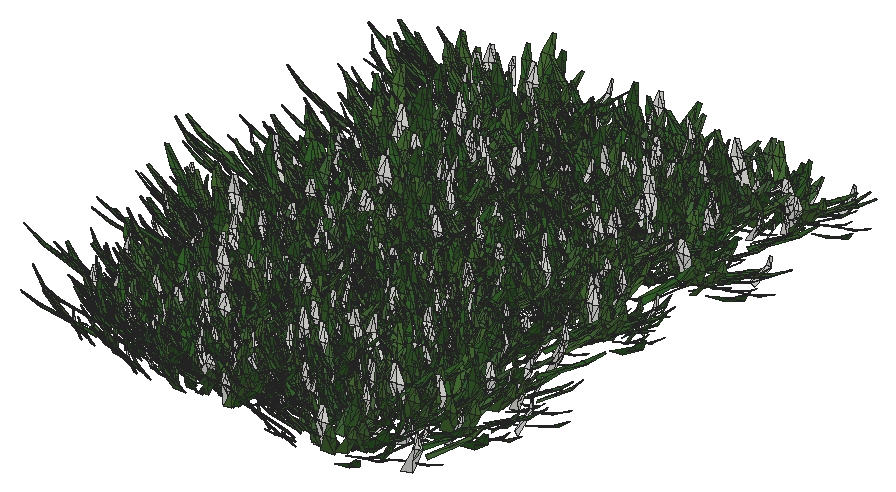
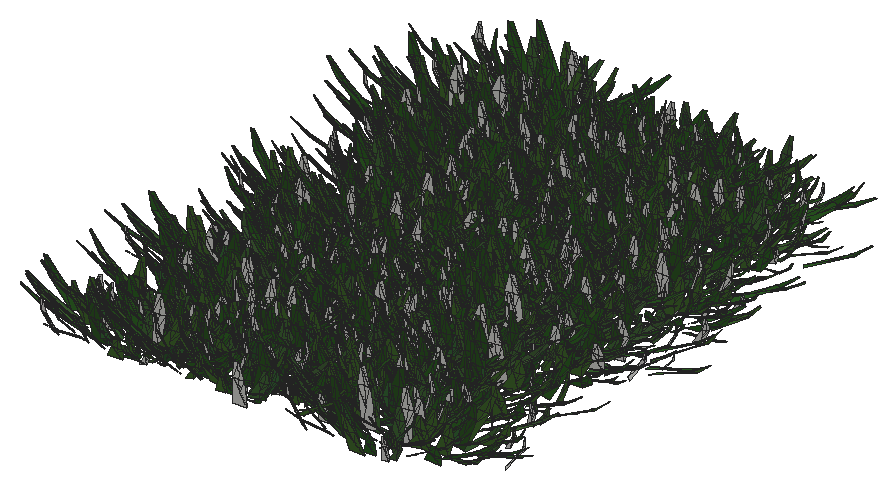
# SketchUp Ruby script. Lengths in inches.
U = 1.inch
M = Sketchup.active_model
def pt(a) = Geom::Point3d.new(a.map { |v| v * U })
def face(e, loops, mat)
  f = e.add_face(loops[0].map { |a| pt(a) })
  loops[1..].each { |l| e.add_face(l.map { |a| pt(a) }).erase! }
  f.material = f.back_material = mat if mat
  f
end
# faces: each face lists its corners as indices into pts; further lists are holes
def faces(e, pts, list, mat = nil) = list.each { |f| face(e, (f[0].is_a?(Array) ? f : [f]).map { |l| l.map { |i| pts[i] } }, mat) }
# xy, xz, yz: faces in a plane at the given z, y or x. An outline is a flat list of corners, or four numbers for a rectangle; further outlines are holes
def ring(l) = l.size == 4 ? [[l[0], l[1]], [l[2], l[1]], [l[2], l[3]], [l[0], l[3]]] : l.each_slice(2).to_a
def flat(e, list, mat, &to3) = list.each { |f| face(e, (f[0].is_a?(Array) ? f : [f]).map { |l| ring(l).map { |u, v| to3.(u, v) } }, mat) }
def xy(e, z, list, mat = nil) = flat(e, list, mat) { |x, y| [x, y, z] }
def xz(e, y, list, mat = nil) = flat(e, list, mat) { |x, z| [x, y, z] }
def yz(e, x, list, mat = nil) = flat(e, list, mat) { |y, z| [x, y, z] }
def lines(e, pts, list) = list.each { |a, b| e.add_line(pt(pts[a]), pt(pts[b])) }
# prism: a flat outline (further loops are holes) pulled along v
def prism(e, loops, v, mat = nil)
  f = face(e, loops, mat); d = Geom::Vector3d.new(v.map { |x| x * U })
  f.pushpull(f.normal.samedirection?(d) ? d.length : -d.length)
end
def box(e, o, s, mat = nil) = prism(e, [[o, [o[0] + s[0], o[1], o[2]], [o[0] + s[0], o[1] + s[1], o[2]], [o[0], o[1] + s[1], o[2]]]], [0, 0, s[2]], mat)
def at(x, y, z, deg = 0) = Geom::Transformation.translation(pt([x, y, z])) * Geom::Transformation.rotation(ORIGIN, Z_AXIS, deg.degrees)
def axes(o, x, y, z) = Geom::Transformation.new([*x, 0, *y, 0, *z, 0, *pt(o).to_a, 1])
def part(name) = M.definitions.add(name)
# library, detail: a bought-in or finely detailed component or shape, given as its bounding box
def library(name, o, s) = part(name).tap { |d| box(d.entities, o, s) }
def detail(e, o, s) = box(e.add_group.entities, o, s)
def put(e, d, t, mat = nil) = e.add_instance(d, t).tap { |i| i.material = mat if mat }
def group(e, t, mat = nil) = e.add_group.tap { |g| g.transformation = t; g.material = mat if mat }.entities
root = M.entities
M.materials.add("Material82").color = [68, 110, 58]
M.materials.add("Material83").color = [48, 90, 38]
M.materials.add("Material84").color = [68, 110, 48]
M.materials.add("Material85").color = [48, 90, 48]
M.materials.add("Material86").color = [58, 110, 58]
M.materials.add("Material87").color = [58, 90, 38]
M.materials.add("Material88").color = [68, 100, 58]
M.materials.add("Material89").color = [48, 100, 38]
c1 = part("grass00")
p = [[-0.6875,0.15,0],[-0.56,0.08,5.52],[-0.04,0.03,2.76],[0.48,-0.02,0],[0.35,-0.02,5.52],[-0.1,-0.14,5.52],
  [-0.12,0.65,8.37],[-0.42,0.65,8.37]]
faces(c1.entities,p,[[0,1,2,3],[3,2,4],[1,5,2],[5,4,2],[1,6,5],[4,5,6],[7,6,1]])
c2 = part("Group16\#1")
put(c2.entities,c1,axes([1.44,-0.61,-0.01],[0.05352,0.12609,0],[-0.10704,0.04543,0.07239],[0.06664,-0.02828,0.11628]),"Material85")
put(c2.entities,c1,axes([0.76,-0.15,-0.01],[0.04676,0.24062,0],[-0.23162,0.04501,0.06642],[0.0652,-0.01267,0.23595]),"Material82")
put(c2.entities,c1,axes([0.79,0.01,-0.01],[-0.00606,0.34651,0],[-0.34381,-0.00602,0.0432],[0.04319,0.00076,0.34386]))
put(c2.entities,c1,axes([1,0.23,-0.01],[-0.07192,0.31144,0],[-0.28722,-0.06632,0.1236],[0.12043,0.02781,0.29478]),"Material84")
put(c2.entities,c1,axes([1.66,0.77,-0.01],[-0.13828,0.29651,0],[-0.21551,-0.1005,0.22471],[0.20365,0.09498,0.23779]),"Material89")
put(c2.entities,c1,axes([0.6875,0.52,-0.01],[-0.18126,0.24051,0],[-0.22746,-0.17142,0.09788],[0.07817,0.05891,0.28481]),"Material84")
put(c2.entities,c1,axes([0.68,0.78,-0.01],[-0.215,0.18688,0],[-0.12385,-0.14248,0.21334],[0.13995,0.16101,0.18878]),"Material82")
put(c2.entities,c1,axes([0.56,1,-0.01],[-0.13756,0.07624,0],[-0.06159,-0.11112,0.0927],[0.04494,0.08108,0.12705]),"Material84")
put(c2.entities,c1,axes([0.2,0.64,-0.01],[-0.23729,0.07254,0],[-0.05711,-0.18681,0.153],[0.04473,0.14632,0.19535]),"Material89")
put(c2.entities,c1,axes([0.0625,0.72,-0.01],[-0.28874,0.02525,0],[-0.02179,-0.24916,0.14647],[0.01276,0.14591,0.25012]),"Material82")
put(c2.entities,c1,axes([-0.08,0.62,-0.01],[-0.34089,-0.04187,0],[0.03255,-0.26504,0.216],[-0.02633,0.21439,0.26703]),"Material89")
put(c2.entities,c1,axes([-0.34,0.98,-0.01],[-0.14314,-0.0493,0],[0.04397,-0.12769,0.06843],[-0.02228,0.0647,0.13505]),"Material89")
put(c2.entities,c1,axes([-0.87,1.45,-0.01],[-0.23488,-0.14114,0],[0.13761,-0.22901,0.06087],[-0.03135,0.05217,0.26717]))
put(c2.entities,c1,axes([-0.72,0.77,-0.01],[-0.14208,-0.13251,0],[0.07209,-0.0773,0.16301],[-0.11118,0.11922,0.1057]),"Material89")
put(c2.entities,c1,axes([-0.62,0.43,-0.01],[-0.14845,-0.21203,0],[0.18654,-0.13061,0.12304],[-0.10079,0.07057,0.22772]),"Material82")
put(c2.entities,c1,axes([-0.68,0.29,-0.01],[-0.13639,-0.32136,0],[0.31723,-0.13464,0.05579],[-0.05136,0.0218,0.34462]),"Material83")
put(c2.entities,c1,axes([-0.64,0.125,-0.01],[-0.0458,-0.23569,0],[0.22124,-0.043,0.08276],[-0.08124,0.01579,0.22538]),"Material86")
put(c2.entities,c1,axes([-1.6,-0.03,-0.01],[0.00576,-0.32897,0],[0.27526,0.00482,0.18018],[-0.18015,-0.00315,0.2753]),"Material84")
put(c2.entities,c1,axes([-1.36,-0.31,-0.01],[0.05718,-0.24765,0],[0.18172,0.04196,0.17267],[-0.16825,-0.03885,0.1865]),"Material89")
put(c2.entities,c1,axes([-1.54,-0.72,-0.01],[0.06537,-0.14017,0],[0.13555,0.06321,0.03939],[-0.0357,-0.01665,0.14956]))
put(c2.entities,c1,axes([-1.19,-0.9,-0.01],[0.09597,-0.12735,0],[0.11214,0.08451,0.07557],[-0.06035,-0.04548,0.14042]),"Material88")
put(c2.entities,c1,axes([-0.47,-0.54,-0.01],[0.11588,-0.10072,0],[0.0618,0.0711,0.12124],[-0.07953,-0.0915,0.0942]))
put(c2.entities,c1,axes([-0.47,-0.84,-0.01],[0.11927,-0.0661,0],[0.06603,0.11913,0.00646],[-0.00313,-0.00565,0.13621]),"Material84")
put(c2.entities,c1,axes([-0.38,-1.24,-0.01],[0.28037,-0.08571,0],[0.0618,0.20215,0.20315],[-0.05939,-0.19428,0.21139]),"Material88")
put(c2.entities,c1,axes([-0.06,-0.66,-0.01],[0.22719,-0.01987,0],[0.01247,0.14255,0.17758],[-0.01547,-0.17691,0.1431]),"Material87")
put(c2.entities,c1,axes([0.11,-0.89,-0.01],[0.14882,0.01828,0],[-0.01058,0.08611,0.12229],[0.01491,-0.12138,0.08676]),"Material85")
put(c2.entities,c1,axes([0.25,-0.72,-0.01],[0.20481,0.07053,0],[-0.06206,0.18022,0.10291],[0.03351,-0.0973,0.1906]),"Material85")
put(c2.entities,c1,axes([0.85,-1.42,-0.01],[0.16481,0.09904,0],[-0.09472,0.15762,0.05616],[0.02893,-0.04814,0.18389]),"Material84")
put(c2.entities,c1,axes([1.01,-1.09,-0.01],[0.21858,0.20385,0],[-0.17495,0.1876,0.15339],[0.10462,-0.11218,0.25652]),"Material89")
put(c2.entities,c1,axes([1.01,-0.71,-0.01],[0.08733,0.12473,0],[-0.06445,0.04512,0.13037],[0.1068,-0.07477,0.07867]),"Material85")
c3 = part("Group15\#1")
put(c3.entities,c2,at(0,0,0))
c4 = part("3darcstudiotree_grass00\#1")
put(c4.entities,c3,at(0,0,0))
put(root,c4,axes([1698.7,940.35,-29.74],[0.55958,-1.81201,0],[3.80263,0.18264,-0.0324],[0.16574,0.00796,1.47946]))
put(root,c4,axes([1684.2,940.68,-29.74],[3.74746,0.48768,0],[-1.05117,1.25627,-0.0401],[-0.08448,0.10096,1.69032]))
put(root,c4,axes([1700.66,941.68,-29.74],[-3.98203,-0.87024,0],[2.1917,-1.55976,-0.02403],[0.066,-0.04697,1.92026]))
put(root,c4,axes([1686.97,941.92,-29.74],[-3.4101,0.33219,0],[-0.86784,-1.38556,-0.03348],[-0.045,-0.07185,1.52035]))
put(root,c4,axes([1675.85,942.55,-29.74],[3.16343,0.45899,0],[-1.51538,1.62437,-0.05896],[-0.12026,0.12891,1.94308]))
put(root,c4,axes([1695.14,942.79,-29.74],[2.81615,0.69239,0],[-1.81737,1.14964,-0.0044],[-0.01183,0.00748,1.30779]))
put(root,c4,axes([1682.83,943.04,-29.74],[3.17869,1.06939,0],[-2.97014,1.37309,-0.05603],[-0.1904,0.08802,1.79617]))
put(root,c4,axes([1683.79,944.17,-29.74],[4.17705,-0.03481,0],[0.09875,1.84286,-0.00824],[0.00079,0.01483,1.59977]))
put(root,c4,axes([1678.98,943.97,-29.74],[-4.39724,-0.41789,0],[0.97106,-1.58919,-0.03666],[0.03598,-0.05889,1.30149]))
put(root,c4,axes([1694.63,945.17,-29.74],[3.16975,0.46707,0],[-1.43384,1.51339,-0.02415],[-0.05301,0.05595,1.92547]))
put(root,c4,axes([1688.77,944.65,-29.74],[-0.72391,1.71321,0],[-3.27988,-0.21555,-0.00349],[-0.01869,-0.00123,1.35435]))
put(root,c4,axes([1698.61,945.14,-29.74],[-2.94402,-0.61655,0],[1.96985,-1.46292,-0.05452],[0.11404,-0.08469,1.404]))
put(root,c4,axes([1688.6,945.91,-29.74],[-3.95806,-0.26007,0],[0.56997,-1.34913,-0.01531],[0.01744,-0.04128,1.80136]))
put(root,c4,axes([1684.06,946.01,-29.74],[-4.52935,0.02332,0],[-0.05756,-1.73901,-0.02897],[-0.00164,-0.04958,1.4344]))
put(root,c4,axes([1701,946.56,-29.74],[-2.23453,-0.97852,0],[2.77364,-0.9851,-0.04825],[0.23755,-0.08437,1.85346]))
put(root,c4,axes([1675.45,946.37,-29.74],[-3.49662,-0.83415,0],[2.45665,-1.60161,-0.00291],[0.00652,-0.00425,1.54121]))
put(root,c4,axes([1694.37,946.48,-29.74],[-3.15856,-0.38514,0],[1.26271,-1.61061,-0.02785],[0.04659,-0.05943,1.81462]))
put(root,c4,axes([1699.63,948.31,-29.74],[1.39356,-1.72752,0],[4.38256,0.54985,-0.00448],[0.02218,0.00278,1.79011]))
put(root,c4,axes([1695.25,948.29,-29.74],[3.28885,0.70173,0],[-2.10741,1.53616,-0.00222],[-0.00511,0.00372,1.6055]))
put(root,c4,axes([1673.45,948.71,-29.74],[1.45525,-1.36358,0],[3.3603,0.55776,-0.00467],[0.02235,0.00371,1.41828]))
put(root,c4,axes([1704.3,949.04,-29.74],[0.57397,-1.69302,0],[4.41794,0.23295,-0.0102],[0.05353,0.00282,1.76846]))
put(root,c4,axes([1676.59,948.57,-29.74],[0.70399,1.48206,0],[-4.34932,0.32132,-0.00799],[-0.0357,0.00264,1.50733]))
put(root,c4,axes([1681.59,949.06,-29.74],[0.05707,-1.33182,0],[4.67038,0.03113,-0.02351],[0.10833,0.00072,1.61343]))
put(root,c4,axes([1688.92,949.375,-29.74],[2.93587,-1.18133,0],[2.75704,1.06566,-0.0131],[0.05816,0.02248,1.79861]))
put(root,c4,axes([1688.45,950.18,-29.74],[0.93986,-1.61608,0],[3.43783,0.31095,-0.013],[0.09422,0.00852,1.96601]))
put(root,c4,axes([1679.29,950.68,-29.74],[-3.07103,-1.30718,0],[3.25603,-1.18973,-0.02123],[0.06738,-0.02462,1.43939]))
put(root,c4,axes([1673.15,950.39,-29.74],[-3.95181,0.01249,0],[-0.03447,-1.69649,-0.00779],[-0.00033,-0.01629,1.71052]))
put(root,c4,axes([1683.02,950.92,-29.74],[-3.14814,-1.33954,0],[3.08708,-1.12839,-0.01903],[0.08494,-0.03105,1.91973]))
put(root,c4,axes([1698.07,950.75,-29.74],[-3.70599,0.79197,0],[-2.20745,-1.60656,-0.0133],[-0.03552,-0.02585,1.94738]))
put(root,c4,axes([1693.7,951.125,-29.74],[-1.513,1.21159,0],[-3.36011,-0.6526,-0.03193],[-0.17356,-0.03371,1.70102]))
put(root,c4,axes([1699.41,952.375,-29.74],[-0.43315,-1.7077,0],[3.80872,-0.15025,-0.05423],[0.31945,-0.0126,1.69842]))
put(root,c4,axes([1678.11,953.12,-29.74],[3.9873,-0.15062,0],[0.35569,1.46445,-0.02913],[0.01977,0.08141,1.9903]))
put(root,c4,axes([1693.89,953.14,-29.74],[3.21716,0.40848,0],[-1.16198,1.42335,-0.048],[-0.09517,0.11657,1.83855]))
put(root,c4,axes([1688.86,953.36,-29.74],[-0.9687,-1.6973,0],[3.99206,-0.35436,-0.03143],[0.1527,-0.01355,1.52743]))
put(root,c4,axes([1703.375,953.78,-29.74],[2.35188,-1.38482,0],[3.12769,0.82614,-0.05113],[0.23612,0.06237,1.56833]))
put(root,c4,axes([1684.1875,953.33,-29.74],[-2.94959,0.77761,0],[-1.85667,-1.09533,-0.00767],[-0.02785,-0.01643,1.63569]))
put(root,c4,axes([1688.73,954.69,-29.74],[-0.43954,-1.59759,0],[3.53501,-0.15126,-0.05057],[0.33495,-0.01433,1.77563]))
put(root,c4,axes([1675.61,955.23,-29.74],[0.98995,-1.43102,0],[4.03348,0.43397,-0.01691],[0.08344,0.00898,1.6028]))
put(root,c4,axes([1695.75,955.49,-29.74],[3.3322,0.38036,0],[-1.11394,1.51777,-0.02015],[-0.03056,0.04163,1.63787]))
put(root,c4,axes([1703.18,955.36,-29.74],[-3.1964,-0.45712,0],[1.21547,-1.32188,-0.00444],[0.00788,-0.00857,1.39182]))
put(root,c4,axes([1682.44,955.57,-29.74],[-1.72626,1.58438,0],[-3.31687,-0.56206,-0.02574],[-0.1159,-0.01964,1.32606]))
put(root,c4,axes([1699.5,956.01,-29.74],[-3.35036,0.87409,0],[-2.07562,-1.23735,-0.03289],[-0.10016,-0.05971,1.55622]))
put(root,c4,axes([1680.99,956.9,-29.74],[2.55829,-1.10547,0],[3.21956,1.15881,-0.03913],[0.13719,0.04938,1.55084]))
put(root,c4,axes([1699.52,957.42,-29.74],[4.04553,0.2871,0],[-0.83462,1.82911,-0.01866],[-0.01606,0.0352,1.717]))
put(root,c4,axes([1672.77,957.74,-29.74],[2.65299,-0.97546,0],[3.20943,1.35758,-0.02398],[0.06395,0.02705,1.37951]))
put(root,c4,axes([1694.84,957.51,-29.74],[-3.75328,0.12847,0],[-0.28677,-1.30306,-0.03872],[-0.02406,-0.10934,1.78675]))
put(root,c4,axes([1677.62,957.78,-29.74],[-3.24632,0.41503,0],[-1.13877,-1.38534,-0.02033],[-0.04358,-0.05301,1.92362]))
put(root,c4,axes([1688.2,958.09,-29.74],[-3.60435,-0.22712,0],[0.60496,-1.49319,-0.01241],[0.00897,-0.02215,1.31731]))
put(root,c4,axes([1689.78,958.9375,-29.74],[1.97331,-1.7001,0],[3.41411,0.61633,-0.04178],[0.21918,0.03957,1.62381]))
put(root,c4,axes([1677.07,959.1,-29.74],[-1.21684,1.60263,0],[-3.24686,-0.38342,-0.04102],[-0.25836,-0.03051,1.67021]))
put(root,c4,axes([1673.92,959.22,-29.74],[-4.06047,-0.30244,0],[0.85134,-1.77769,-0.03943],[0.03436,-0.07175,1.61444]))
put(root,c4,axes([1692.15,959.59,-29.74],[3.0128,0.96923,0],[-2.26467,1.09486,-0.0073],[-0.03331,0.01611,1.93831]))
put(root,c4,axes([1698.23,959.93,-29.74],[-2.43541,-1.16543,0],[2.64027,-0.85812,-0.03867],[0.17422,-0.05662,1.49724]))
put(root,c4,axes([1681.1875,960.5,-29.74],[-3.18803,-0.40221,0],[1.38309,-1.70502,-0.00535],[0.00805,-0.00992,1.67969]))
put(root,c4,axes([1700.23,961.28,-29.74],[-2.79186,-1.03231,0],[2.26214,-0.95152,-0.04465],[0.21173,-0.08906,1.71883]))
put(root,c4,axes([1672.59,961.18,-29.74],[-1.54224,1.54277,0],[-3.96225,-0.61604,-0.03242],[-0.18554,-0.02885,1.96368]))
put(root,c4,axes([1682.01,961.25,-29.74],[-2.16052,1.42464,0],[-3.02099,-0.71254,-0.01081],[-0.04852,-0.01144,1.38013]))
put(root,c4,axes([1687.95,961.87,-29.74],[3.59479,1.11581,0],[-2.65109,1.32837,-0.01986],[-0.0739,0.03703,1.93312]))
put(root,c4,axes([1677.32,962.29,-29.74],[4.36912,-0.54802,0],[1.07763,1.33621,-0.00335],[0.00554,0.00687,1.45436]))
put(root,c4,axes([1694.48,962.06,-29.74],[0.73987,1.59354,0],[-4.44696,0.32112,-0.04305],[-0.22862,0.01651,1.82947]))
put(root,c4,axes([1671.25,963.26,-29.74],[3.29517,0.70525,0],[-2.24642,1.63243,-0.00178],[-0.00323,0.00235,1.34491]))
put(root,c4,axes([1698.74,963.76,-29.74],[-3.56566,-0.8896,0],[2.32838,-1.45148,-0.01513],[0.04457,-0.02778,1.79885]))
put(root,c4,axes([1677.8,963.88,-29.74],[1.39223,1.25256,0],[-3.795,0.65605,-0.01361],[-0.06427,0.01111,1.60179]))
put(root,c4,axes([1681.58,964.22,-29.74],[1.97793,1.10174,0],[-3.47293,0.96971,-0.06047],[-0.20758,0.05796,1.34144]))
put(root,c4,axes([1692.2,964.26,-29.74],[-2.92804,-0.86099,0],[2.52273,-1.33432,-0.01853],[0.05328,-0.02818,1.52144]))
put(root,c4,axes([1687.53,964.65,-29.74],[-1.63823,-1.36099,0],[3.49292,-0.65391,-0.00409],[0.01763,-0.0033,1.3842]))
put(root,c4,axes([1687.4,965.68,-29.74],[2.36777,-1.25491,0],[3.70344,1.08678,-0.00846],[0.02737,0.00803,1.39582]))
put(root,c4,axes([1699.68,965.51,-29.74],[-3.34111,0.18713,0],[-0.56421,-1.56678,-0.00819],[-0.00515,-0.01431,1.3463]))
put(root,c4,axes([1694.92,965.92,-29.74],[0.58066,1.77085,0],[-3.90665,0.19923,-0.04685],[-0.26361,0.01344,1.67517]))
put(root,c4,axes([1681.99,966.68,-29.74],[-4.52964,-0.09494,0],[0.22898,-1.69903,-0.02618],[0.00745,-0.05528,1.73378]))
put(root,c4,axes([1676.98,966.96,-29.74],[-2.17136,1.02025,0],[-2.89421,-0.95801,-0.02769],[-0.1122,-0.03714,1.49833]))
put(root,c4,axes([1687.71,968.42,-29.74],[3.08639,0.66231,0],[-1.76537,1.27948,-0.04213],[-0.09869,0.07153,1.35679]))
put(root,c4,axes([1703.73,968.78,-29.74],[1.1756,-1.47793,0],[3.44657,0.42639,-0.02865],[0.17647,0.02183,1.74795]))
put(root,c4,axes([1673.27,968.89,-29.74],[4.53982,0.21063,0],[-0.49544,1.66085,-0.02625],[-0.01899,0.06364,1.96735]))
put(root,c4,axes([1681.33,969.01,-29.74],[0.12157,-1.62148,0],[4.39568,0.05126,-0.0158],[0.08264,0.00096,1.72451]))
put(root,c4,axes([1696.05,968.9,-29.74],[-1.04498,-1.27032,0],[4.0983,-0.52433,-0.01227],[0.0665,-0.00851,1.83962]))
put(root,c4,axes([1701.2,968.89,-29.74],[2.22198,1.23467,0],[-3.2898,0.92081,-0.0048],[-0.02055,0.00575,1.58899]))
put(root,c4,axes([1675.96,969.1875,-29.74],[3.78243,-0.20016,0],[0.50434,1.48226,-0.04419],[0.03105,0.09126,1.50171]))
put(root,c4,axes([1694.88,969.88,-29.74],[3.7109,-0.91214,0],[2.11846,1.34044,-0.04378],[0.13838,0.08756,1.79394]))
put(root,c4,axes([1687.1,970.45,-29.74],[3.96894,-0.58875,0],[1.33194,1.3965,-0.01237],[0.02838,0.02976,1.84855]))
put(root,c4,axes([1679.47,970.52,-29.74],[0.11291,-1.83708,0],[4.52912,0.0433,-0.04883],[0.22915,0.00219,1.59403]))
put(root,c4,axes([1672.41,970.91,-29.74],[4.70379,-0.18713,0],[0.44198,1.72795,-0.01121],[0.00446,0.01743,1.30781]))
put(root,c4,axes([1684.33,971.21,-29.74],[2.20471,-1.56419,0],[3.09714,0.67895,-0.02727],[0.12975,0.02844,1.44583]))
put(root,c4,axes([1698.57,971.18,-29.74],[2.778,0.72584,0],[-2.53603,1.50959,-0.00365],[-0.00789,0.0047,1.34685]))
put(root,c4,axes([1694.58,972.25,-29.74],[3.34228,0.13265,0],[-0.43082,1.68835,-0.00091],[-0.00041,0.00162,1.45853]))
put(root,c4,axes([1700.29,972.03,-29.74],[3.42042,0.9713,0],[-2.12433,1.16348,-0.02682],[-0.10129,0.05548,1.76121]))
put(root,c4,axes([1688.93,972.11,-29.74],[3.30561,0.92504,0],[-2.54174,1.41264,-0.05586],[-0.15004,0.08339,1.52805]))
put(root,c4,axes([1682.4375,973.27,-29.74],[2.97087,-0.63768,0],[1.76888,1.28171,-0.04084],[0.13668,0.09904,1.94165]))
put(root,c4,axes([1677.56,973.18,-29.74],[-4.25587,0.04591,0],[-0.1089,-1.57017,-0.04984],[-0.00682,-0.0984,1.49526]))
put(root,c4,axes([1677.53,974.41,-29.74],[0.66389,-1.49509,0],[4.57403,0.31589,-0.04237],[0.23153,0.01599,1.93074]))
put(root,c4,axes([1671.9375,974.33,-29.74],[-0.08871,1.46443,0],[-4.0853,-0.03849,-0.0357],[-0.16722,-0.00158,1.43525]))
put(root,c4,axes([1681.67,974.75,-29.74],[-4.65824,0.34825,0],[-0.74927,-1.55877,-0.04366],[-0.04609,-0.09588,1.70895]))
put(root,c4,axes([1689.17,975.62,-29.74],[-1.5733,-1.53629,0],[3.8056,-0.60614,-0.01424],[0.06159,-0.00981,1.43479]))
put(root,c4,axes([1699.71,975.46,-29.74],[-3.34476,-0.15722,0],[0.48645,-1.60959,-0.01308],[0.00826,-0.02735,1.64432]))
put(root,c4,axes([1692.5,975.79,-29.74],[-3.6982,-1.11774,0],[2.6803,-1.37926,-0.01589],[0.04062,-0.0209,1.38765]))
put(root,c4,axes([1677.82,977.21,-29.74],[3.97153,-0.13343,0],[0.30373,1.40602,-0.01096],[0.00672,0.03109,1.93666]))
put(root,c4,axes([1694.16,977.11,-29.74],[1.27309,1.64144,0],[-4.4392,0.53549,-0.03143],[-0.12353,0.0149,1.42994]))
put(root,c4,axes([1684.0625,977.33,-29.74],[-2.73035,-0.81396,0],[2.55013,-1.33042,-0.03674],[0.11326,-0.05909,1.62045]))
put(root,c4,axes([1697.98,977.35,-29.74],[-0.26231,1.84263,0],[-3.30675,-0.07321,-0.00552],[-0.03272,-0.00072,1.47331]))
put(root,c4,axes([1686.58,977.54,-29.74],[-4.55367,0.27818,0],[-0.67765,-1.72528,-0.03016],[-0.02264,-0.05764,1.62739]))
put(root,c4,axes([1675.7,978.96,-29.74],[2.00913,-1.08398,0],[3.65765,1.05439,-0.0361],[0.15471,0.0446,1.80295]))
put(root,c4,axes([1696.12,979.02,-29.74],[1.02841,-1.31305,0],[3.38391,0.41221,-0.03395],[0.18437,0.02246,1.50895]))
put(root,c4,axes([1689.77,978.55,-29.74],[-3.47148,-0.32447,0],[1.09042,-1.81447,-0.00987],[0.00954,-0.01587,1.48448]))
put(root,c4,axes([1699.84,979.17,-29.74],[3.21897,1.19921,0],[-3.23164,1.34914,-0.01632],[-0.04651,0.01942,1.46423]))
put(root,c4,axes([1681.42,979.78,-29.74],[3.35413,-0.63199,0],[1.61191,1.33051,-0.01719],[0.04506,0.03719,1.70421]))
put(root,c4,axes([1697.62,980.94,-29.74],[3.19452,-0.59612,0],[1.46474,1.2208,-0.01286],[0.03129,0.02608,1.45976]))
put(root,c4,axes([1690.45,981.03,-29.74],[4.44722,-0.53115,0],[1.26492,1.64719,-0.03542],[0.04521,0.05887,1.44036]))
put(root,c4,axes([1703.92,981.01,-29.74],[0.90068,-1.41561,0],[4.53027,0.44829,-0.03647],[0.13709,0.01357,1.35653]))
put(root,c4,axes([1678.58,981.27,-29.74],[4.35154,-0.63119,0],[1.42423,1.52711,-0.01984],[0.04228,0.04533,1.90869]))
put(root,c4,axes([1692.17,981.38,-29.74],[-4.1478,0.13224,0],[-0.279,-1.36104,-0.02584],[-0.01399,-0.06822,1.74304]))
put(root,c4,axes([1684.49,982.21,-29.74],[1.55533,-1.52655,0],[4.26431,0.67573,-0.03894],[0.20513,0.0325,1.95573]))
put(root,c4,axes([1672.42,982.24,-29.74],[1.46562,-1.72266,0],[4.03529,0.53396,-0.04434],[0.25483,0.03372,1.93394]))
put(root,c4,axes([1679.12,983.45,-29.74],[0.94741,-1.42267,0],[3.73003,0.38633,-0.03356],[0.18091,0.01874,1.61101]))
put(root,c4,axes([1695.15,983.51,-29.74],[3.53019,1.19751,0],[-2.61374,1.19838,-0.04839],[-0.15514,0.07113,1.47711]))
put(root,c4,axes([1700.28,983.24,-29.74],[-2.66899,1.32243,0],[-3.00544,-0.94339,-0.02078],[-0.10429,-0.03273,1.84714]))
put(root,c4,axes([1681.09,984.29,-29.74],[3.44825,-0.26897,0],[0.66516,1.32629,-0.00259],[0.00332,0.00662,1.70099]))
put(root,c4,axes([1689.9,984.23,-29.74],[1.7248,1.72946,0],[-3.94677,0.61218,-0.01805],[-0.10059,0.0156,1.90362]))
put(root,c4,axes([1699.39,985.43,-29.74],[4.2125,0.29861,0],[-0.756,1.65872,-0.00017],[-0.00017,0.00037,1.78268]))
put(root,c4,axes([1676.72,985.46,-29.74],[3.77678,0.27869,0],[-0.6902,1.45473,-0.00485],[-0.00557,0.01174,1.75633]))
put(root,c4,axes([1695.61,986,-29.74],[1.40396,-1.3283,0],[3.66211,0.60201,-0.02113],[0.09939,0.01634,1.51549]))
put(root,c4,axes([1682.33,985.83,-29.74],[-3.60203,-0.72226,0],[1.64221,-1.27378,-0.05096],[0.13667,-0.10601,1.60728]))
put(root,c4,axes([1690.61,986.68,-29.74],[2.99585,-0.78884,0],[2.43675,1.4393,-0.03164],[0.10153,0.05997,1.90074]))
put(root,c4,axes([1672.92,987.37,-29.74],[3.00061,-1.20381,0],[2.59687,1.00673,-0.02297],[0.10061,0.039,1.67632]))
put(root,c4,axes([1678.99,987.7,-29.74],[2.81234,1.34734,0],[-2.81254,0.91306,-0.01155],[-0.05543,0.018,1.69697]))
put(root,c4,axes([1689.86,988.21,-29.74],[3.0975,-0.44176,0],[1.39811,1.52468,-0.04794],[0.07202,0.07854,1.36124]))
put(root,c4,axes([1692.0625,988.2,-29.74],[2.38875,-0.89777,0],[2.38741,0.98797,-0.03437],[0.15253,0.06312,1.66865]))
put(root,c4,axes([1699.8125,987.84,-29.74],[-4.04939,0.05434,0],[-0.15117,-1.75202,-0.01213],[-0.00231,-0.02678,1.86653]))
put(root,c4,axes([1683.32,988.4375,-29.74],[-1.19412,-1.34448,0],[3.1862,-0.44013,-0.02961],[0.14836,-0.02049,1.34337]))
put(root,c4,axes([1698.625,989.65,-29.74],[-2.58541,-0.85496,0],[2.80483,-1.31917,-0.0116],[0.03194,-0.01502,1.40225]))
put(root,c4,axes([1677.01,989.56,-29.74],[-3.45253,0.27622,0],[-0.72182,-1.40321,-0.01756],[-0.02267,-0.04407,1.76676]))
put(root,c4,axes([1695.29,990.17,-29.74],[0.99609,-1.23763,0],[4.45512,0.55768,-0.04397],[0.17141,0.02146,1.43296]))
put(root,c4,axes([1688.2,989.76,-29.74],[-4.42879,-0.33071,0],[0.76141,-1.58586,-0.02653],[0.02727,-0.05679,1.69452]))
put(root,c4,axes([1682.7,990.76,-29.74],[-3.59651,-0.44623,0],[1.25179,-1.56915,-0.00258],[0.00335,-0.0042,1.35273]))
put(root,c4,axes([1682.91,991.78,-29.74],[3.47707,-0.28838,0],[0.88445,1.65855,-0.04208],[0.03591,0.06734,1.3356]))
put(root,c4,axes([1671.72,991.65,-29.74],[0.85595,1.34318,0],[-4.39323,0.43542,-0.04255],[-0.19043,0.01887,1.5668]))
put(root,c4,axes([1692.76,992.3125,-29.74],[0.38467,-1.72776,0],[3.7527,0.12994,-0.02351],[0.1369,0.00474,1.65028]))
put(root,c4,axes([1689.02,991.85,-29.74],[-3.45853,-0.30921,0],[0.875,-1.52216,-0.03754],[0.05438,-0.09459,1.94323]))
put(root,c4,axes([1701.53,992.52,-29.74],[-1.62678,1.3546,0],[-3.70168,-0.6914,-0.05633],[-0.31213,-0.0583,1.88219]))
put(root,c4,axes([1675.55,992.54,-29.74],[-2.26736,0.9467,0],[-3.26135,-1.21483,-0.01576],[-0.0639,-0.0238,1.87507]))
put(root,c4,axes([1690.25,994.12,-29.74],[4.2542,-0.55295,0],[1.2277,1.46904,-0.0158],[0.03318,0.0397,1.97161]))
put(root,c4,axes([1677.01,994.43,-29.74],[0.78455,-1.57227,0],[3.87046,0.30038,-0.05061],[0.32766,0.02543,1.95081]))
put(root,c4,axes([1694.125,993.85,-29.74],[-4.20928,0.13814,0],[-0.29813,-1.41294,-0.01346],[-0.00713,-0.03379,1.72106]))
put(root,c4,axes([1703.8,994.56,-29.74],[1.41685,-1.43454,0],[3.76136,0.57778,-0.0174],[0.0698,0.01072,1.30214]))
put(root,c4,axes([1700.3125,993.97,-29.74],[-3.91283,-0.66077,0],[1.78522,-1.64415,-0.00601],[0.01088,-0.01002,1.5624]))
